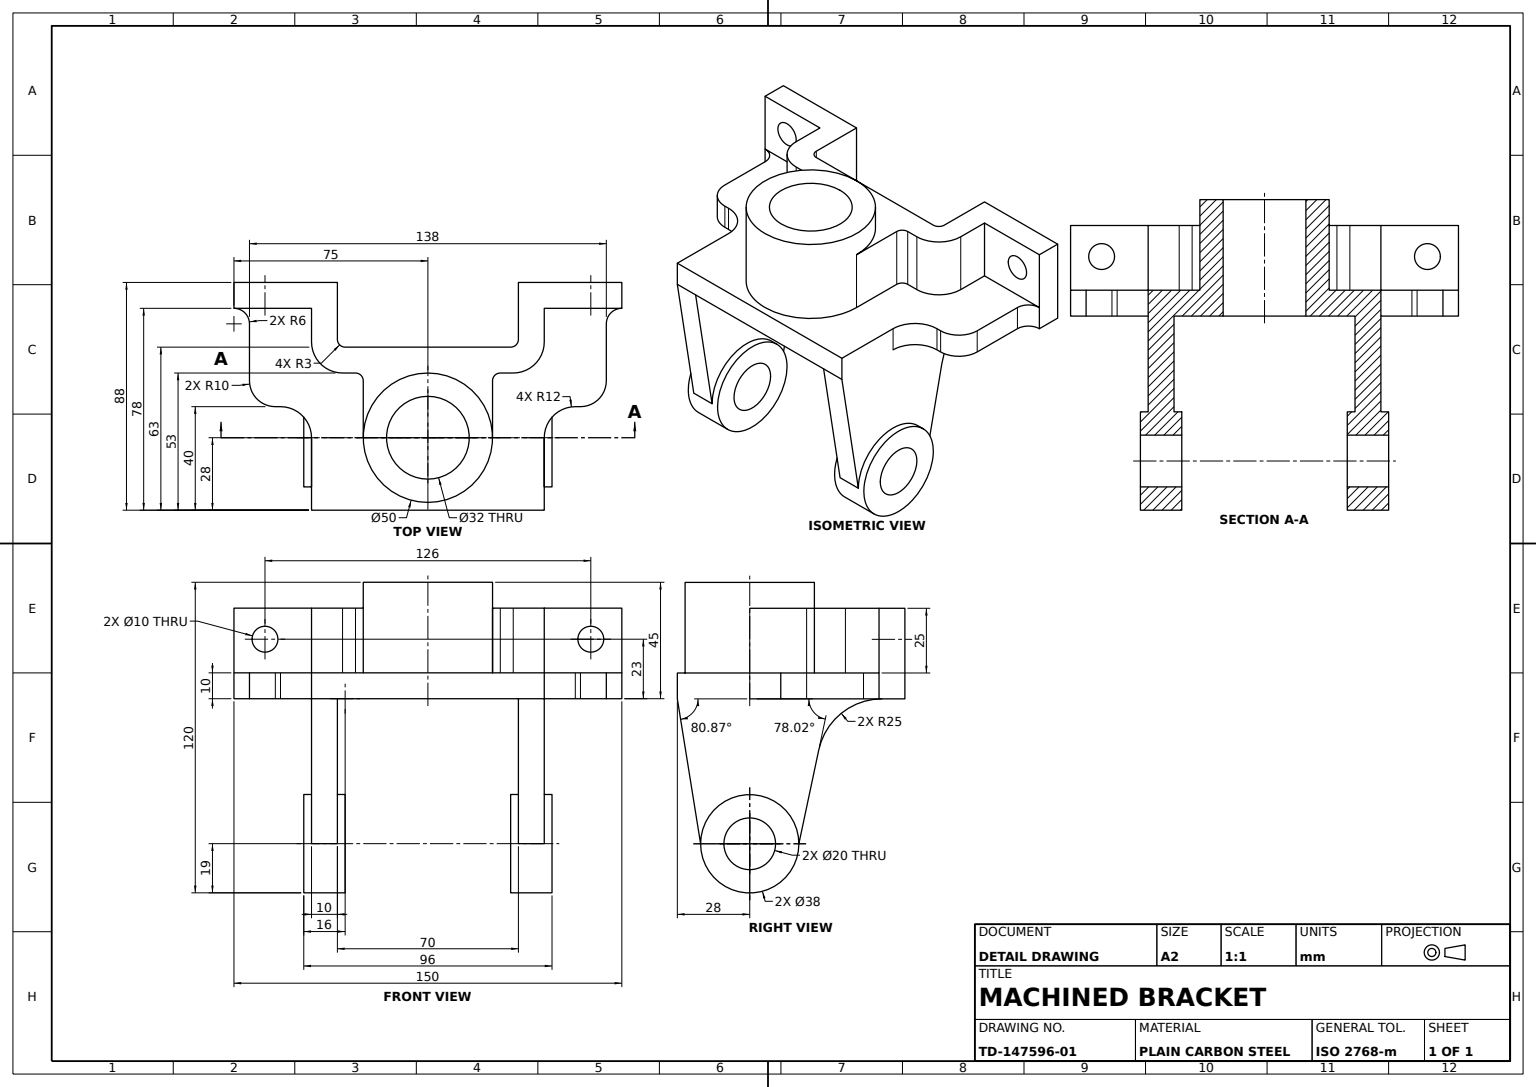
solid
v1 (32,-56,10)
v2 (48,-56,10)
e1 v1 v2 LINE
v3 (32,-56,-10)
e2 v3 v1 CIRCLE(AX(P(32,-56,0),D(1,0,0),D(0,0,-1)),10)
v4 (48,-56,-10)
e3 v3 v4 LINE
e4 v4 v2 CIRCLE(AX(P(48,-56,0),D(1,0,0),D(0,0,-1)),10)
face CYL(AX(P(32,-56,0),D(1,0,0),D(0,0,-1)),10) rev [-e1 -e2 e3 e4]
v5 (45,-19.812395,-26.676159)
v6 (45,-56,-19)
e5 v5 v6 LINE
v7 (35,-56,-19)
e6 v7 v6 LINE
v8 (35,-19.812395,-26.676159)
e7 v8 v7 LINE
e8 v8 v5 LINE
face PLANE(AX(P(35,-6.268014,-29.549209),D(0,0.207504208,0.978234125),D(0,-0.978234125,0.207504208))) rev [e5 -e6 -e7 e8]
v9 (28,35,-25)
v10 (25,35,-22)
e9 v9 v10 CIRCLE(AX(P(28,35,-22),D(0,1,0),D(0,0,1)),3)
v11 (25,10,-22)
e10 v10 v11 LINE
v12 (28,10,-25)
e11 v12 v11 CIRCLE(AX(P(28,10,-22),D(0,1,0),D(0,0,1)),3)
e12 v9 v12 LINE
face CYL(AX(P(28,35,-22),D(0,-1,0),D(0,0,-1)),3) rev [e9 e10 -e11 -e12]
v13 (58,23,-50)
v14 (68,23,-50)
e13 v13 v14 CIRCLE(AX(P(63,23,-50),D(0,0,1),D(1,0,0)),5)
e14 v14 v13 CIRCLE(AX(P(63,23,-50),D(0,0,1),D(1,0,0)),5)
v15 (75,35,-50)
v16 (75,10,-50)
e15 v15 v16 LINE
v17 (45,35,-50)
e16 v15 v17 LINE
v18 (45,10,-50)
e17 v17 v18 LINE
e18 v16 v18 LINE
face PLANE(AX(P(0,35,-50),D(0,0,1),D(1,0,0))) [-e13 -e14] [-e15 e16 e17 -e18]
v19 (-25,35,-22)
v20 (-25,10,-22)
e19 v19 v20 LINE
v21 (-25,10,0)
e20 v21 v20 LINE
v22 (-25,35,0)
e21 v22 v21 LINE
e22 v22 v19 LINE
face PLANE(AX(P(-25,35,0),D(-1,0,0),D(0,0,1))) [e19 -e20 -e21 e22]
v23 (-58,23,-50)
v24 (-68,23,-50)
e23 v23 v24 CIRCLE(AX(P(-63,23,-50),D(0,0,1),D(1,0,0)),5)
v25 (-68,23,-60)
e24 v25 v24 LINE
v26 (-58,23,-60)
e25 v25 v26 CIRCLE(AX(P(-63,23,-60),D(0,0,-1),D(-1,0,0)),5)
e26 v26 v23 LINE
face CYL(AX(P(-63,23,-95),D(0,0,1),D(1,0,0)),5) rev [e23 -e24 e25 e26]
e27 v1 v3 CIRCLE(AX(P(32,-56,0),D(1,0,0),D(0,0,-1)),10)
v27 (32,-56,19)
v28 (32,-56,-19)
e28 v27 v28 CIRCLE(AX(P(32,-56,0),D(1,0,0),D(0,0,-1)),19)
e29 v28 v27 CIRCLE(AX(P(32,-56,0),D(1,0,0),D(0,0,-1)),19)
face PLANE(AX(P(32,0,0),D(1,0,0),D(0,0,-1))) rev [e2 e27] [-e28 -e29]
v29 (75,0,-50)
e30 v16 v29 LINE
v30 (75,0,-60)
e31 v30 v29 LINE
v31 (75,35,-60)
e32 v31 v30 LINE
e33 v31 v15 LINE
face PLANE(AX(P(75,35,0),D(1,0,0),D(0,0,-1))) [e15 e30 -e31 -e32 e33]
v32 (59,10,-12)
v33 (59,0,-12)
e34 v32 v33 LINE
v34 (69,0,-22)
e35 v34 v33 CIRCLE(AX(P(59,0,-22),D(0,-1,0),D(0,0,1)),10)
v35 (69,10,-22)
e36 v35 v34 LINE
e37 v35 v32 CIRCLE(AX(P(59,10,-22),D(0,-1,0),D(0,0,1)),10)
face CYL(AX(P(59,10,-22),D(0,-1,0),D(0,0,-1)),10) [e34 -e35 -e36 e37]
v36 (-45,-19.812395,-26.676159)
v37 (-45,-56,-19)
e38 v36 v37 LINE
v38 (-45,-56,19)
e39 v38 v37 CIRCLE(AX(P(-45,-56,0),D(-1,0,0),D(0,0,1)),19)
v39 (-45,0,28)
e40 v39 v38 LINE
v40 (-45,10,28)
e41 v40 v39 LINE
v41 (-45,10,0)
e42 v40 v41 LINE
v42 (-45,0,0)
e43 v41 v42 LINE
v43 (-45,0,-51.132012)
e44 v43 v42 LINE
e45 v43 v36 CIRCLE(AX(P(-45,-25,-51.132012),D(1,0,0),D(0,0,1)),25)
face PLANE(AX(P(-45,10,28),D(-1,0,0),D(0,0,1))) [e38 -e39 -e40 -e41 e42 e43 -e44 e45]
v44 (-28,35,-25)
v45 (-33,35,-25)
e46 v44 v45 LINE
v46 (-33,10,-25)
e47 v45 v46 LINE
v47 (-28,10,-25)
e48 v47 v46 LINE
e49 v44 v47 LINE
face PLANE(AX(P(0,35,-25),D(0,0,1),D(1,0,0))) [e46 e47 -e48 -e49]
v48 (35,0,-51.132012)
e50 v48 v8 CIRCLE(AX(P(35,-25,-51.132012),D(1,0,0),D(0,0,-1)),25)
v49 (45,0,-51.132012)
e51 v49 v48 LINE
e52 v5 v49 CIRCLE(AX(P(45,-25,-51.132012),D(-1,0,0),D(0,0,-1)),25)
face CYL(AX(P(35,-25,-51.132012),D(-1,0,0),D(0,0,1)),25) rev [-e50 -e51 -e52 -e8]
v50 (-35,0,28)
e53 v50 v39 LINE
v51 (-35,-56,19)
e54 v51 v38 LINE
e55 v50 v51 LINE
face PLANE(AX(P(-35,-4.386696,27.294995),D(0,0.158678095,-0.987330371),D(0,0.987330371,0.158678095))) rev [e53 e40 -e54 -e55]
v52 (-48,-56,-10)
v53 (-48,-56,10)
e56 v52 v53 CIRCLE(AX(P(-48,-56,0),D(-1,0,0),D(0,0,1)),10)
e57 v53 v52 CIRCLE(AX(P(-48,-56,0),D(-1,0,0),D(0,0,1)),10)
v54 (-48,-56,19)
v55 (-48,-56,-19)
e58 v54 v55 CIRCLE(AX(P(-48,-56,0),D(-1,0,0),D(0,0,1)),19)
e59 v55 v54 CIRCLE(AX(P(-48,-56,0),D(-1,0,0),D(0,0,1)),19)
face PLANE(AX(P(-48,-56,0),D(-1,0,0),D(0,0,1))) [-e56 -e57] [e58 e59]
e60 v37 v55 LINE
e61 v38 v54 LINE
face CYL(AX(P(-32,-56,0),D(-1,0,0),D(0,0,1)),19) [e60 -e58 -e61 e39]
v56 (0,10,25)
e62 v21 v56 CIRCLE(AX(P(0,10,0),D(0,1,0),D(0,0,1)),25)
e63 v20 v47 CIRCLE(AX(P(-28,10,-22),D(0,1,0),D(0,0,1)),3)
v57 (-45,10,-37)
e64 v46 v57 CIRCLE(AX(P(-33,10,-37),D(0,-1,0),D(0,0,1)),12)
v58 (-45,10,-50)
e65 v57 v58 LINE
v59 (-75,10,-50)
e66 v58 v59 LINE
v60 (-69,10,-44)
e67 v60 v59 CIRCLE(AX(P(-75,10,-44),D(0,1,0),D(0,0,-1)),6)
v61 (-69,10,-22)
e68 v61 v60 LINE
v62 (-59,10,-12)
e69 v62 v61 CIRCLE(AX(P(-59,10,-22),D(0,-1,0),D(0,0,-1)),10)
v63 (-57,10,-12)
e70 v63 v62 LINE
e71 v41 v63 CIRCLE(AX(P(-57,10,0),D(0,1,0),D(0,0,1)),12)
v64 (45,10,28)
e72 v64 v40 LINE
v65 (45,10,0)
e73 v65 v64 LINE
v66 (57,10,-12)
e74 v66 v65 CIRCLE(AX(P(57,10,0),D(0,1,0),D(0,0,-1)),12)
e75 v32 v66 LINE
v67 (69,10,-44)
e76 v67 v35 LINE
e77 v16 v67 CIRCLE(AX(P(75,10,-44),D(0,1,0),D(0,0,-1)),6)
v68 (45,10,-37)
e78 v18 v68 LINE
v69 (33,10,-25)
e79 v68 v69 CIRCLE(AX(P(33,10,-37),D(0,-1,0),D(0,0,1)),12)
e80 v69 v12 LINE
v70 (25,10,0)
e81 v11 v70 LINE
e82 v56 v70 CIRCLE(AX(P(0,10,0),D(0,1,0),D(0,0,1)),25)
face PLANE(AX(P(-57,10,0),D(0,1,0),D(0,0,1))) [-e62 e20 e63 e48 e64 e65 e66 -e67 -e68 -e69 -e70 -e71 -e42 -e72 -e73 -e74 -e75 -e37 -e76 -e77 e18 e78 e79 e80 e11 e81 -e82]
v71 (-69,0,-44)
v72 (-75,0,-50)
e83 v71 v72 CIRCLE(AX(P(-75,0,-44),D(0,1,0),D(0,0,-1)),6)
e84 v60 v71 LINE
e85 v59 v72 LINE
face CYL(AX(P(-75,10,-44),D(0,-1,0),D(0,0,-1)),6) rev [-e83 -e84 e67 e85]
v73 (68,23,-60)
e86 v73 v14 LINE
v74 (58,23,-60)
e87 v73 v74 CIRCLE(AX(P(63,23,-60),D(0,0,-1),D(-1,0,0)),5)
e88 v74 v13 LINE
face CYL(AX(P(63,23,-95),D(0,0,1),D(1,0,0)),5) rev [e13 -e86 e87 e88]
v75 (48,-56,-19)
v76 (48,-56,19)
e89 v75 v76 CIRCLE(AX(P(48,-56,0),D(1,0,0),D(0,0,-1)),19)
e90 v6 v75 LINE
v77 (45,-56,19)
e91 v6 v77 CIRCLE(AX(P(45,-56,0),D(1,0,0),D(0,0,-1)),19)
e92 v77 v76 LINE
face CYL(AX(P(32,-56,0),D(1,0,0),D(0,0,-1)),19) [-e89 -e90 e91 e92]
v78 (-35,35,-38)
v79 (-35,0,-38)
e93 v78 v79 LINE
v80 (-35,0,-51.132012)
e94 v80 v79 LINE
v81 (-35,0,-60)
e95 v81 v80 LINE
v82 (-35,35,-60)
e96 v82 v81 LINE
e97 v82 v78 LINE
face PLANE(AX(P(-35,35,0),D(1,0,0),D(0,0,-1))) [e93 -e94 -e95 -e96 e97]
v83 (-32,35,-35)
e98 v78 v83 CIRCLE(AX(P(-32,35,-38),D(0,1,0),D(0,0,1)),3)
v84 (-32,0,-35)
e99 v83 v84 LINE
e100 v79 v84 CIRCLE(AX(P(-32,0,-38),D(0,1,0),D(0,0,1)),3)
face CYL(AX(P(-32,35,-38),D(0,-1,0),D(0,0,-1)),3) rev [e98 e99 -e100 -e93]
v85 (-32,-56,10)
v86 (-32,-56,-10)
e101 v85 v86 CIRCLE(AX(P(-32,-56,0),D(-1,0,0),D(0,0,1)),10)
e102 v85 v53 LINE
e103 v86 v52 LINE
face CYL(AX(P(-32,-56,0),D(-1,0,0),D(0,0,1)),10) rev [-e101 e102 e57 -e103]
v87 (45,35,-37)
e104 v87 v68 LINE
e105 v17 v87 LINE
face PLANE(AX(P(45,35,0),D(1,0,0),D(0,0,-1))) [e104 -e78 -e17 e105]
v88 (35,0,-60)
e106 v48 v88 LINE
e107 v88 v30 LINE
v89 (69,0,-44)
e108 v29 v89 CIRCLE(AX(P(75,0,-44),D(0,1,0),D(0,0,-1)),6)
e109 v89 v34 LINE
v90 (57,0,-12)
e110 v33 v90 LINE
v91 (45,0,0)
e111 v90 v91 CIRCLE(AX(P(57,0,0),D(0,1,0),D(0,0,-1)),12)
e112 v91 v49 LINE
face PLANE(AX(P(0,0,0),D(0,1,0),D(0,0,1))) rev [e51 e106 e107 e31 e108 e109 e35 e110 e111 e112]
e113 v28 v7 LINE
v92 (35,-56,19)
e114 v27 v92 LINE
e115 v7 v92 CIRCLE(AX(P(35,-56,0),D(1,0,0),D(0,0,-1)),19)
face CYL(AX(P(32,-56,0),D(1,0,0),D(0,0,-1)),19) [-e113 e29 e114 -e115]
v93 (35,35,-38)
v94 (35,35,-60)
e116 v93 v94 LINE
e117 v94 v88 LINE
v95 (35,0,-38)
e118 v95 v48 LINE
e119 v93 v95 LINE
face PLANE(AX(P(35,35,0),D(-1,0,0),D(0,0,1))) [e116 e117 -e106 -e118 -e119]
v96 (0,45,25)
v97 (0,45,-25)
e120 v96 v97 CIRCLE(AX(P(0,45,0),D(0,1,0),D(0,0,1)),25)
e121 v96 v56 LINE
v98 (25,35,0)
e122 v98 v70 LINE
v99 (0,35,-25)
e123 v98 v99 CIRCLE(AX(P(0,35,0),D(0,1,0),D(0,0,1)),25)
e124 v97 v99 LINE
face CYL(AX(P(0,45,0),D(0,-1,0),D(0,0,-1)),25) [-e120 e121 e82 -e122 e123 -e124]
v100 (-32,-56,19)
v101 (-32,-56,-19)
e125 v100 v101 CIRCLE(AX(P(-32,-56,0),D(-1,0,0),D(0,0,1)),19)
e126 v101 v100 CIRCLE(AX(P(-32,-56,0),D(-1,0,0),D(0,0,1)),19)
e127 v86 v85 CIRCLE(AX(P(-32,-56,0),D(-1,0,0),D(0,0,1)),10)
face PLANE(AX(P(-32,0,0),D(-1,0,0),D(0,0,1))) rev [-e125 -e126] [e101 e127]
v102 (35,0,28)
e128 v102 v50 LINE
e129 v79 v50 LINE
v103 (32,0,-35)
e130 v84 v103 LINE
e131 v103 v95 CIRCLE(AX(P(32,0,-38),D(0,1,0),D(0,0,1)),3)
e132 v102 v95 LINE
v104 (0,0,16)
v105 (0,0,-16)
e133 v104 v105 CIRCLE(AX(P(0,0,0),D(0,1,0),D(0,0,1)),16)
e134 v105 v104 CIRCLE(AX(P(0,0,0),D(0,1,0),D(0,0,1)),16)
face PLANE(AX(P(0,0,0),D(0,1,0),D(0,0,1))) rev [e128 -e129 e100 e130 e131 -e132] [e133 e134]
e135 v99 v22 CIRCLE(AX(P(0,35,0),D(0,1,0),D(0,0,1)),25)
e136 v97 v96 CIRCLE(AX(P(0,45,0),D(0,1,0),D(0,0,1)),25)
face CYL(AX(P(0,45,0),D(0,-1,0),D(0,0,-1)),25) [e124 e135 e21 e62 -e121 -e136]
e137 v2 v4 CIRCLE(AX(P(48,-56,0),D(1,0,0),D(0,0,-1)),10)
e138 v76 v75 CIRCLE(AX(P(48,-56,0),D(1,0,0),D(0,0,-1)),19)
face PLANE(AX(P(48,-56,0),D(1,0,0),D(0,0,-1))) [-e137 -e4] [e138 e89]
v106 (0,45,-16)
v107 (0,45,16)
e139 v106 v107 CIRCLE(AX(P(0,45,0),D(0,1,0),D(0,0,1)),16)
e140 v107 v104 LINE
e141 v106 v105 LINE
face CYL(AX(P(0,45,0),D(0,-1,0),D(0,0,-1)),16) rev [e139 e140 -e134 -e141]
v108 (-35,-56,-19)
e142 v51 v108 CIRCLE(AX(P(-35,-56,0),D(-1,0,0),D(0,0,1)),19)
e143 v100 v51 LINE
e144 v101 v108 LINE
face CYL(AX(P(-32,-56,0),D(-1,0,0),D(0,0,1)),19) [-e142 -e143 e125 e144]
e145 v67 v89 LINE
face CYL(AX(P(75,10,-44),D(0,-1,0),D(0,0,-1)),6) rev [e145 -e108 -e30 e77]
e146 v80 v43 LINE
v109 (-35,-19.812395,-26.676159)
e147 v109 v80 CIRCLE(AX(P(-35,-25,-51.132012),D(-1,0,0),D(0,0,1)),25)
e148 v36 v109 LINE
face CYL(AX(P(0,-25,-51.132012),D(-1,0,0),D(0,0,1)),25) rev [-e146 -e147 -e148 -e45]
v110 (-57,0,-12)
v111 (-59,0,-12)
e149 v110 v111 LINE
e150 v63 v110 LINE
e151 v62 v111 LINE
face PLANE(AX(P(-57,10,-12),D(0,0,1),D(1,0,0))) [-e149 -e150 e70 e151]
e152 v107 v106 CIRCLE(AX(P(0,45,0),D(0,1,0),D(0,0,1)),16)
face CYL(AX(P(0,45,0),D(0,-1,0),D(0,0,-1)),16) rev [-e140 e152 e141 -e133]
e153 v26 v25 CIRCLE(AX(P(-63,23,-60),D(0,0,-1),D(-1,0,0)),5)
v112 (-75,0,-60)
e154 v112 v81 LINE
v113 (-75,35,-60)
e155 v113 v112 LINE
e156 v113 v82 LINE
face PLANE(AX(P(0,35,-60),D(0,0,-1),D(-1,0,0))) [-e153 -e25] [-e154 -e155 e156 e96]
v114 (33,35,-25)
e157 v114 v69 LINE
e158 v114 v9 LINE
face PLANE(AX(P(0,35,-25),D(0,0,1),D(1,0,0))) [e12 -e80 -e157 e158]
e159 v24 v23 CIRCLE(AX(P(-63,23,-50),D(0,0,1),D(1,0,0)),5)
face CYL(AX(P(-63,23,-95),D(0,0,1),D(1,0,0)),5) rev [-e26 e153 e24 e159]
v115 (32,35,-35)
e160 v115 v103 LINE
e161 v115 v93 CIRCLE(AX(P(32,35,-38),D(0,1,0),D(0,0,1)),3)
face CYL(AX(P(32,35,-38),D(0,-1,0),D(0,0,-1)),3) rev [e119 -e131 -e160 e161]
e162 v108 v37 LINE
face CYL(AX(P(-32,-56,0),D(-1,0,0),D(0,0,1)),19) [-e144 e126 e143 e54 e61 -e59 -e60 -e162]
e163 v94 v31 LINE
e164 v74 v73 CIRCLE(AX(P(63,23,-60),D(0,0,-1),D(-1,0,0)),5)
face PLANE(AX(P(0,35,-60),D(0,0,-1),D(-1,0,0))) [-e117 e163 e32 -e107] [-e87 -e164]
v116 (-45,35,-50)
e165 v116 v58 LINE
v117 (-75,35,-50)
e166 v116 v117 LINE
e167 v117 v59 LINE
face PLANE(AX(P(0,35,-50),D(0,0,1),D(1,0,0))) [-e23 -e159] [-e66 -e165 e166 e167]
e168 v10 v98 LINE
e169 v87 v114 CIRCLE(AX(P(33,35,-37),D(0,-1,0),D(0,0,1)),12)
e170 v83 v115 LINE
e171 v117 v113 LINE
v118 (-45,35,-37)
e172 v118 v116 LINE
e173 v45 v118 CIRCLE(AX(P(-33,35,-37),D(0,-1,0),D(0,0,1)),12)
e174 v19 v44 CIRCLE(AX(P(-28,35,-22),D(0,1,0),D(0,0,1)),3)
face PLANE(AX(P(0,35,0),D(0,1,0),D(0,0,1))) [-e135 -e123 -e168 -e9 -e158 -e169 -e105 -e16 -e33 -e163 -e116 -e161 -e170 -e98 -e97 -e156 -e171 -e166 -e172 -e173 -e46 -e174 -e22]
e175 v102 v92 LINE
e176 v92 v77 LINE
v119 (45,0,28)
e177 v119 v77 LINE
e178 v119 v102 LINE
face PLANE(AX(P(35,-4.386696,27.294995),D(0,-0.158678095,0.987330371),D(0,-0.987330371,-0.158678095))) [e175 e176 -e177 e178]
face CYL(AX(P(32,-56,0),D(1,0,0),D(0,0,-1)),19) [e113 e6 e90 -e138 -e92 -e176 -e114 e28]
face CYL(AX(P(-32,-56,0),D(-1,0,0),D(0,0,1)),10) rev [e103 e56 -e102 -e127]
e179 v109 v108 LINE
face PLANE(AX(P(-35,0,0),D(-1,0,0),D(0,0,1))) rev [e94 e129 e55 e142 -e179 e147]
e180 v65 v91 LINE
e181 v64 v119 LINE
face PLANE(AX(P(45,10,28),D(1,0,0),D(0,0,-1))) [-e5 e52 -e112 -e180 e73 e181 e177 -e91]
e182 v72 v112 LINE
face PLANE(AX(P(-75,35,0),D(-1,0,0),D(0,0,1))) [-e85 -e167 e171 e155 -e182]
v120 (-69,0,-22)
e183 v61 v120 LINE
e184 v111 v120 CIRCLE(AX(P(-59,0,-22),D(0,-1,0),D(0,0,-1)),10)
face CYL(AX(P(-59,10,-22),D(0,-1,0),D(0,0,-1)),10) [-e151 e69 e183 -e184]
face PLANE(AX(P(-35,-6.268014,-29.549209),D(0,-0.207504208,-0.978234125),D(0,0.978234125,-0.207504208))) [e148 e179 e162 -e38]
e185 v66 v90 LINE
face PLANE(AX(P(57,10,-12),D(0,0,1),D(1,0,0))) [-e34 e75 e185 -e110]
face CYL(AX(P(63,23,-95),D(0,0,1),D(1,0,0)),5) rev [-e88 e164 e86 e14]
e186 v42 v110 CIRCLE(AX(P(-57,0,0),D(0,1,0),D(0,0,1)),12)
e187 v120 v71 LINE
face PLANE(AX(P(0,0,0),D(0,1,0),D(0,0,1))) rev [e83 e182 e154 e95 e146 e44 e186 e149 e184 e187]
face PLANE(AX(P(0,45,0),D(0,1,0),D(0,0,1))) [e136 e120] [-e152 -e139]
face CYL(AX(P(32,-56,0),D(1,0,0),D(0,0,-1)),10) rev [e1 e137 -e3 -e27]
e188 v118 v57 LINE
face CYL(AX(P(-33,35,-37),D(0,-1,0),D(0,0,-1)),12) [e188 -e64 -e47 e173]
face PLANE(AX(P(-45,10,28),D(0,0,1),D(1,0,0))) [-e178 -e181 e72 e41 -e53 -e128]
face PLANE(AX(P(25,35,0),D(1,0,0),D(0,0,-1))) [-e10 e168 e122 -e81]
face CYL(AX(P(57,10,0),D(0,-1,0),D(0,0,-1)),12) rev [e180 -e111 -e185 e74]
face PLANE(AX(P(0,35,-35),D(0,0,-1),D(-1,0,0))) [e170 e160 -e130 -e99]
face PLANE(AX(P(69,10,-22),D(1,0,0),D(0,0,-1))) [-e109 -e145 e76 e36]
face CYL(AX(P(33,35,-37),D(0,-1,0),D(0,0,-1)),12) [e157 -e79 -e104 e169]
face CYL(AX(P(-28,35,-22),D(0,-1,0),D(0,0,-1)),3) rev [e174 e49 -e63 -e19]
face PLANE(AX(P(-69,10,-22),D(-1,0,0),D(0,0,1))) [e84 -e187 -e183 e68]
face PLANE(AX(P(-45,35,0),D(-1,0,0),D(0,0,1))) [e172 e165 -e65 -e188]
face CYL(AX(P(-57,10,0),D(0,-1,0),D(0,0,-1)),12) rev [-e186 -e43 e71 e150]
face PLANE(AX(P(35,0,0),D(1,0,0),D(0,0,-1))) rev [e7 e115 -e175 e132 e118 e50]
